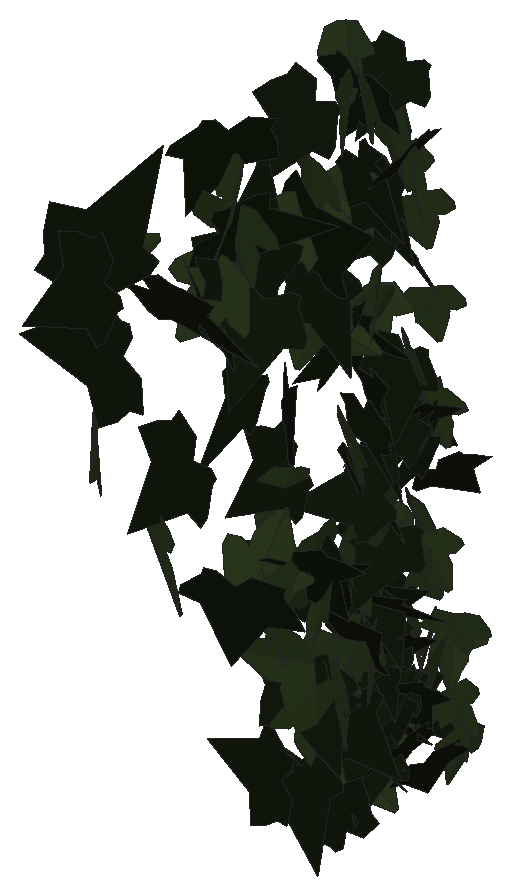
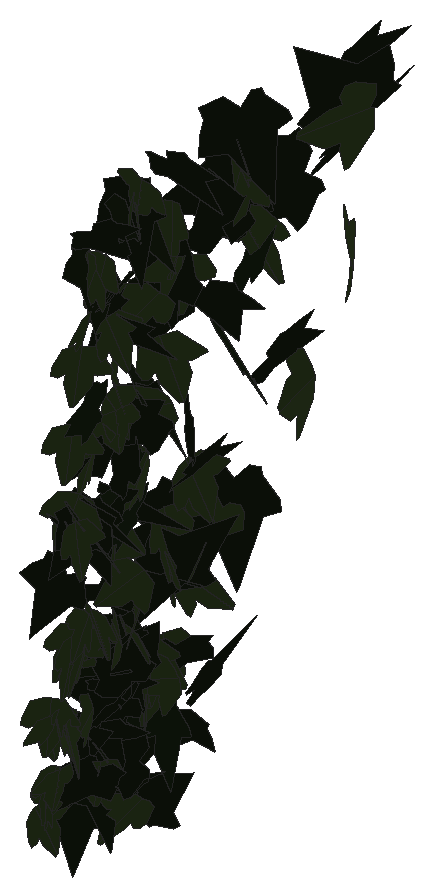
# SketchUp Ruby script. Lengths in inches.
U = 1.inch
M = Sketchup.active_model
def pt(a) = Geom::Point3d.new(a.map { |v| v * U })
def face(e, loops, mat)
  f = e.add_face(loops[0].map { |a| pt(a) })
  loops[1..].each { |l| e.add_face(l.map { |a| pt(a) }).erase! }
  f.material = f.back_material = mat if mat
  f
end
# faces: each face lists its corners as indices into pts; further lists are holes
def faces(e, pts, list, mat = nil) = list.each { |f| face(e, (f[0].is_a?(Array) ? f : [f]).map { |l| l.map { |i| pts[i] } }, mat) }
# xy, xz, yz: faces in a plane at the given z, y or x. An outline is a flat list of corners, or four numbers for a rectangle; further outlines are holes
def ring(l) = l.size == 4 ? [[l[0], l[1]], [l[2], l[1]], [l[2], l[3]], [l[0], l[3]]] : l.each_slice(2).to_a
def flat(e, list, mat, &to3) = list.each { |f| face(e, (f[0].is_a?(Array) ? f : [f]).map { |l| ring(l).map { |u, v| to3.(u, v) } }, mat) }
def xy(e, z, list, mat = nil) = flat(e, list, mat) { |x, y| [x, y, z] }
def xz(e, y, list, mat = nil) = flat(e, list, mat) { |x, z| [x, y, z] }
def yz(e, x, list, mat = nil) = flat(e, list, mat) { |y, z| [x, y, z] }
def lines(e, pts, list) = list.each { |a, b| e.add_line(pt(pts[a]), pt(pts[b])) }
# prism: a flat outline (further loops are holes) pulled along v
def prism(e, loops, v, mat = nil)
  f = face(e, loops, mat); d = Geom::Vector3d.new(v.map { |x| x * U })
  f.pushpull(f.normal.samedirection?(d) ? d.length : -d.length)
end
def box(e, o, s, mat = nil) = prism(e, [[o, [o[0] + s[0], o[1], o[2]], [o[0] + s[0], o[1] + s[1], o[2]], [o[0], o[1] + s[1], o[2]]]], [0, 0, s[2]], mat)
def at(x, y, z, deg = 0) = Geom::Transformation.translation(pt([x, y, z])) * Geom::Transformation.rotation(ORIGIN, Z_AXIS, deg.degrees)
def axes(o, x, y, z) = Geom::Transformation.new([*x, 0, *y, 0, *z, 0, *pt(o).to_a, 1])
def part(name) = M.definitions.add(name)
# library, detail: a bought-in or finely detailed component or shape, given as its bounding box
def library(name, o, s) = part(name).tap { |d| box(d.entities, o, s) }
def detail(e, o, s) = box(e.add_group.entities, o, s)
def put(e, d, t, mat = nil) = e.add_instance(d, t).tap { |i| i.material = mat if mat }
def group(e, t, mat = nil) = e.add_group.tap { |g| g.transformation = t; g.material = mat if mat }.entities
root = M.entities
M.materials.add("efeu1").color = [18, 25, 13]
M.materials.add("efeu2").color = [43, 57, 29]
c1 = part("ivyleaf_10")
p = [[0,0.5,-0.03],[-0.0625,2.02,-0.43],[-0.19,2.01,-0.46],[-0.54,1.05,-0.29],[-0.52,0.625,-0.18],[-0.83,0.76,-0.28],
  [-1.16,0.64,-0.33],[-1.15,0.33,-0.24],[-0.77,-0.39,0.02],[-0.3,-0.51,0.16],[0.04,-0.48,0.23],[-0.02,2.01,-0.4375],
  [-0.06,2.01,-0.43],[0.04,-0.49,0.23],[0.67,-0.49,0.14],[1.38,0.36,-0.2],[1.375,0.51,-0.24],[0.81,0.65,-0.19],
  [0.62,0.59,-0.15],[0.6,1.09,-0.28],[0.5,1.23,-0.31]]
faces(c1.entities,p,[[0,1,2,3,4,5,6,7,8,9,10],[11,12,0,13,14,15,16,17,18,19,20]],"efeu2")
c2 = part("ivyleaf_9")
p = [[1.54,2.16,1.25],[1.36,2.04,1.19],[-0.21,0.99,0.68],[-0.71,1.11,0.82],[-0.85,0.86,0.67],[-0.8,0.17,0.21],
  [-0.9,-0.01,0.1],[-0.67,-0.16,-0.02],[-0.08,-0.08,-0.05],[-0.03,-0.6,-0.4],[0.65,-0.88,-0.66],[0.83,-0.6,-0.49],
  [1.29,-0.42,-0.43],[1.8125,-0.07,-0.26],[1.21,0.44,0.15]]
faces(c2.entities,p,[[0,1,2,3,4,5,6,7,8,9,10,11,12,13,14]],"efeu1")
put(root,c1,axes([600.42,135.75,192.35],[-0.57947,-0.09583,-0.54206],[0.53378,0.09451,-0.58732],[0.13452,-0.78783,-0.00451]))
put(root,c2,axes([601.29,134.13,183.22],[0.15939,-0.00668,0.8756],[-0.77177,0.41934,0.14369],[-0.41362,-0.785,0.0693]))
put(root,c2,axes([600.17,135.93,185.94],[0.73929,-0.09917,0.34207],[0.33915,-0.04465,-0.74591],[0.10876,0.81337,0.00076]))
put(root,c1,axes([600.875,136.26,201.3],[-0.11468,-0.73234,0.25084],[-0.01013,-0.25213,-0.74076],[0.77404,-0.11181,0.02747]))
put(root,c1,axes([600.48,135.19,206.09],[0.75673,-0.04398,0.3091],[0.30983,0.00602,-0.75768],[0.03843,0.8174,0.02221]))
put(root,c2,axes([600.82,132.46,194.53],[-0.32847,-0.57411,0.70321],[-0.20623,-0.68108,-0.65238],[0.88406,-0.37219,0.10909]))
put(root,c1,axes([600.52,135.61,184.05],[0.26824,0.56099,0.52859],[0.23902,0.47156,-0.62176],[-0.7328,0.35917,-0.00931]))
put(root,c1,axes([600.5625,124.19,203.86],[0.0746,-0.00351,-1.25714],[0.50326,1.15412,0.02664],[1.15202,-0.50395,0.06977]))
put(root,c1,axes([600.97,132.1,194.31],[-0.17849,-0.85958,0.319],[0.01065,-0.32691,-0.87494],[0.9168,-0.16355,0.07227]))
put(root,c1,axes([600.34,134.18,188.08],[-0.33958,0.10618,-0.76231],[0.72104,-0.24756,-0.35568],[-0.26922,-0.79696,0.00892]))
put(root,c2,axes([600.39,134.69,197.75],[0.7539,0.15262,0.31025],[0.30319,0.06595,-0.76919],[-0.1662,0.81258,0.00416]))
put(root,c2,axes([601.1875,129.375,206],[0.12559,0.81604,-0.69572],[-0.07243,-0.69242,-0.82525],[-1.06991,0.14266,-0.0258]))
put(root,c1,axes([600.51,134.69,201.83],[0.49246,0.4161,0.51638],[0.38042,0.34959,-0.64449],[-0.5432,0.62205,0.01679]))
put(root,c2,axes([601.39,132.66,190.91],[0.16136,0.04894,0.94365],[-0.92224,-0.20032,0.16809],[0.20577,-0.93616,0.01336]))
put(root,c1,axes([600.89,135.32,189.9375],[0.75204,-0.43582,0.00601],[0.01492,0.01376,-0.86898],[0.4356,0.75194,0.01939]))
put(root,c1,axes([600.87,136.04,198.04],[0.30519,0.6869,-0.11948],[-0.05319,-0.1071,-0.75163],[-0.69518,0.30974,0.00506]))
put(root,c2,axes([601.36,133.27,186.28],[-0.19484,0.94153,0.12857],[-0.07206,0.11622,-0.96034],[-0.94753,-0.20245,0.0466]))
put(root,c1,axes([600.87,138.97,186.45],[0.12127,0.66909,-0.01265],[-0.00008,-0.01284,-0.67999],[-0.66921,0.12125,-0.00221]))
put(root,c2,axes([601.27,134.74,205.34],[0.58647,0.27011,-0.77571],[-0.72255,-0.28365,-0.64505],[-0.39064,0.93017,0.02856]))
put(root,c2,axes([600.67,132.57,195.53],[-0.17798,0.33647,0.88831],[0.14761,-0.88299,0.36404],[0.93836,0.20272,0.11123]))
put(root,c2,axes([601.41,134.7,204.93],[-0.50561,0.68441,-0.28331],[0.01783,-0.33167,-0.83306],[-0.74052,-0.47529,0.17338]))
put(root,c1,axes([600.45,134.44,197.9],[-0.31329,-0.15336,-0.74743],[0.75783,0.03143,-0.3241],[0.08874,-0.80983,0.12897]))
put(root,c1,axes([600.5,124.83,198.99],[-0.08943,0.09935,-1.22983],[0.473,-1.13609,-0.12617],[-1.13957,-0.47935,0.04414]))
put(root,c1,axes([600.85,136.95,185.85],[0.43736,0.59441,0.03481],[0.01938,0.02896,-0.73798],[-0.59511,0.43779,0.00155]))
put(root,c1,axes([601.24,133.2,199.09],[-0.64986,-0.57022,0.32563],[-0.14012,-0.32717,-0.85254],[0.64152,-0.64908,0.14365]))
put(root,c1,axes([601.09,137.72,194.52],[-0.11861,-0.72719,-0.02028],[0.00854,0.01915,-0.73678],[0.72742,-0.1188,0.00535]))
put(root,c1,axes([600.84,132.8125,202.08],[0.65597,0.72367,0.01641],[0.01062,0.01252,-0.97672],[-0.72378,0.65605,0.00054]))
put(root,c2,axes([600.57,137.42,199.07],[0.6371,-0.42672,0.06495],[0.04307,-0.05237,-0.76655],[0.42948,0.63826,-0.01947]))
put(root,c2,axes([600.8,124.2,204.12],[-0.46686,-0.24231,1.14678],[0.97881,0.59845,0.52493],[-0.64477,1.08393,-0.03346]))
put(root,c2,axes([601.43,135.5,200.95],[-0.82481,-0.21666,0.16799],[-0.14614,-0.10316,-0.85057],[0.23195,-0.8354,0.06146]))
put(root,c2,axes([600.74,136.28,187.96],[0.16956,-0.80811,-0.09241],[-0.02675,0.08881,-0.82567],[0.81294,0.17148,-0.0079]))
put(root,c1,axes([601.03,137.5,191.24],[-0.6172,0.34973,-0.07002],[0.05498,-0.04498,-0.70929],[-0.3524,-0.61953,0.01197]))
put(root,c1,axes([601.03,136.81,191.15],[0.67928,-0.29894,-0.04096],[-0.036,0.01989,-0.74214],[0.29958,0.68023,0.0037]))
put(root,c1,axes([601.3,128.95,201.88],[1.02623,-0.09184,-0.47066],[-0.46604,0.07092,-1.02999],[0.11298,1.12678,0.02647]))
put(root,c2,axes([600.46,135.91,188.8],[0.11426,-0.18914,0.75301],[0.74962,-0.1713,-0.15677],[0.20215,0.74212,0.15573]))
put(root,c1,axes([601.05,134.63,190.83],[-0.5381,0.68938,0.05134],[-0.01734,0.05158,-0.87434],[-0.69107,-0.53808,-0.01804]))
put(root,c1,axes([601.12,138.03,187.44],[0.3224,-0.60247,-0.07417],[-0.03645,0.06462,-0.68331],[0.60593,0.32445,-0.00164]))
put(root,c1,axes([601.0625,137.66,190.09],[-0.49479,0.50117,-0.00216],[0.00138,-0.00168,-0.70426],[-0.50117,-0.49479,0.0002]))
put(root,c2,axes([600.875,135.87,184.78],[-0.28621,-0.78529,0.08726],[0.16267,-0.14939,-0.81083],[0.7732,-0.25925,0.20289]))
put(root,c1,axes([601.13,133.75,187.9],[-0.31715,-0.75146,-0.30111],[0.10381,0.28298,-0.81553],[0.80286,-0.33344,-0.0135]))
put(root,c2,axes([601.21,136.72,204.87],[-0.55941,-0.57491,0.05908],[-0.054,-0.02987,-0.80196],[0.57541,-0.56172,-0.01783]))
put(root,c2,axes([600.53,135.18,185.34],[0.64128,-0.34646,0.28615],[0.25479,-0.13038,-0.72886],[0.37013,0.69002,0.00596]))
put(root,c2,axes([601.05,128.04,196.68],[-0.25506,-0.76369,0.73671],[-0.22915,-0.70017,-0.80515],[1.03608,-0.34287,0.00328]))
put(root,c1,axes([601.17,135.78,198.25],[0.05644,-0.71724,0.38027],[0.0236,-0.37958,-0.71944],[0.81147,0.06092,-0.00553]))
put(root,c2,axes([601.24,136.27,186.82],[-0.63447,-0.50927,-0.0238],[0.02074,0.01218,-0.81357],[0.5094,-0.6348,0.00348]))
put(root,c1,axes([600.74,136.14,190.14],[-0.05555,0.12773,-0.75309],[0.40276,-0.63668,-0.13769],[-0.64903,-0.40603,-0.02099]))
put(root,c2,axes([601.21,135.91,188.39],[-0.59629,-0.57435,-0.02227],[0.0133,0.0183,-0.82791],[0.57463,-0.59642,-0.00395]))
put(root,c1,axes([601.44,132.7,203.59],[-0.86133,0.29022,0.30649],[-0.31064,0.0357,-0.9068],[-0.28578,-0.91354,0.06193]))
put(root,c2,axes([600.85,137.07,185.87],[0.0484,-0.29496,-0.71405],[0.08231,0.71335,-0.28909],[0.76818,-0.05785,0.07596]))
put(root,c1,axes([600.96,137.34,187.98],[-0.40273,0.44585,-0.38218],[0.22974,-0.30685,-0.60007],[-0.54042,-0.4627,0.0297]))
put(root,c2,axes([601.45,132.61,205.53],[-0.93032,-0.26697,-0.1007],[0.09403,0.03737,-0.96782],[0.26939,-0.93501,-0.00993]))
put(root,c2,axes([601.7,133.67,198.1],[-0.67645,0.66652,0.01684],[-0.00823,0.01564,-0.94963],[-0.66668,-0.67648,-0.00536]))
put(root,c1,axes([600.76,126.79,195.3],[-0.682,0.68808,-0.743],[0.54477,-0.50584,-0.96849],[-0.85365,-0.87253,-0.02446]))
put(root,c2,axes([601.48,130.14,198.4],[-0.95246,0.29765,-0.41369],[0.39082,-0.13621,-0.99781],[-0.3271,-1.02945,0.01241]))
put(root,c2,axes([600.86,129.35,200.36],[-0.20453,-0.30982,1.0056],[0.21481,-1.01514,-0.26907],[1.03008,0.15018,0.25578]))
put(root,c1,axes([600.9375,130.98,191.95],[0.81918,0.43956,-0.3696],[0.31755,0.18979,0.92952],[0.47852,-0.87843,0.01588]))
put(root,c2,axes([600.74,135.65,195.75],[0.05873,-0.15285,0.76619],[0.3896,-0.66027,-0.16158],[0.67722,0.39311,0.02651]))
put(root,c2,axes([601.27,130.96,200.27],[-0.80788,-0.56282,-0.29022],[0.24835,0.15116,-0.98445],[0.58251,-0.84501,0.0172]))
put(root,c1,axes([600.98,134.72,204.91],[0.30645,-0.58251,0.55429],[0.42777,-0.38417,-0.64023],[0.68086,0.50355,0.15277]))
put(root,c1,axes([601.09,131.35,191.47],[-0.40241,0.84864,-0.31541],[0.1653,-0.27049,-0.93867],[-0.89014,-0.43388,-0.03172]))
put(root,c1,axes([601.39,134.83,205.19],[-0.67626,0.58131,0.08761],[-0.11445,0.0008,-0.88872],[-0.57663,-0.68191,0.07364]))
put(root,c1,axes([601.56,134.14,188.55],[-0.58002,-0.65861,0.2129],[-0.15332,-0.14862,-0.87745],[0.67497,-0.59972,-0.01636]))
put(root,c1,axes([601.36,137.25,200.53],[-0.51434,-0.57058,-0.10471],[0.08601,0.06339,-0.76789],[0.5737,-0.52105,0.02124]))
put(root,c2,axes([601.55,129.33,192.52],[0.69017,0.64815,-0.68048],[-0.49855,-0.46316,-0.9468],[-0.79662,0.85139,0.00298]))
put(root,c1,axes([601.26,137.04,201.88],[-0.22898,0.74611,-0.10082],[0.04723,-0.09094,-0.78024],[-0.75141,-0.23308,-0.01832]))
put(root,c2,axes([601.64,136,184.87],[-0.11842,0.79962,-0.14954],[0.02993,-0.14673,-0.8083],[-0.81293,-0.12188,-0.00798]))
put(root,c2,axes([601.51,131.125,186.05],[0.10503,-0.94989,-0.2167],[0.15393,-0.19904,0.94709],[-0.96206,-0.13554,0.12788]))
put(root,c2,axes([601.83,136.38,194.58],[-0.79579,0.02715,0.13407],[-0.13433,-0.00566,-0.79619],[-0.02583,-0.80698,0.0101]))
put(root,c2,axes([601.05,135.82,189.8],[0.09431,-0.81585,-0.18626],[0.1084,0.19777,-0.81138],[0.82979,0.06689,0.12716]))
put(root,c1,axes([601.48,129.2,203.75],[-1.12996,0.05466,-0.05608],[0.05636,0.00448,-1.13126],[-0.05437,-1.13134,-0.00719]))
put(root,c2,axes([601.65,136.59,194.52],[0.00213,0.65958,-0.47998],[0.00441,-0.47998,-0.65957],[-0.81573,-0.00087,-0.00482]))
put(root,c2,axes([601.51,135.43,187.94],[0.35174,0.77528,0.01543],[-0.02705,0.0292,-0.85055],[-0.77496,0.35086,0.0367]))
put(root,c1,axes([601.79,133.54,187.19],[0.23558,-0.29083,-0.85323],[-0.39433,0.75978,-0.36786],[0.81061,0.45413,0.06902]))
put(root,c1,axes([602.18,131.01,189.84],[0.26175,-0.01114,-1.02215],[-0.97591,0.31122,-0.2533],[0.30415,1.00819,0.0669]))
put(root,c2,axes([601.14,135.02,202.66],[0.46531,-0.625,-0.33915],[-0.1702,0.29563,-0.77833],[0.69042,0.4941,0.03669]))
put(root,c2,axes([601.82,136.1,186.32],[-0.74386,0.29825,-0.1157],[0.08906,-0.08822,-0.79997],[-0.30726,-0.74762,0.04824]))
put(root,c1,axes([601.55,137.45,197.72],[-0.59397,-0.46268,-0.06511],[0.05369,0.03703,-0.7529],[0.46414,-0.59638,0.00376]))
put(root,c1,axes([601.59,132.59,192.51],[-0.0302,-0.91844,-0.1147],[0.01392,0.11429,-0.91888],[0.92547,-0.0317,0.01008]))
put(root,c2,axes([601.59,129.81,201.69],[-0.57177,-0.56786,0.81892],[0.62656,0.52933,0.80452],[-0.77493,0.84697,0.04626]))
put(root,c2,axes([601.05,135.13,189.45],[0.79554,0.14562,0.3072],[0.24781,0.2868,-0.77769],[-0.23275,0.80312,0.22202]))
put(root,c1,axes([601.14,136.71,203.27],[0.54375,-0.38918,0.43163],[0.47411,-0.04483,-0.63768],[0.33613,0.69279,0.20121]))
put(root,c2,axes([601.47,136.125,186.41],[0.59064,0.53904,-0.10921],[-0.09387,-0.0591,-0.7994],[-0.54192,0.59774,0.01944]))
put(root,c1,axes([601.24,135.58,198.93],[0.4779,-0.45427,0.49056],[0.38114,-0.31033,-0.65866],[0.54932,0.61052,0.03022]))
put(root,c2,axes([601.19,132.68,188.26],[-0.06617,-0.79037,-0.52122],[0.14853,0.50735,-0.7882],[0.93503,-0.13652,0.08832]))
put(root,c1,axes([601.61,135.91,203.13],[-0.76893,0.19423,-0.00204],[0.00202,-0.00033,-0.79308],[-0.19423,-0.76893,-0.00017]))
put(root,c2,axes([601.34,135.35,201.96],[0.31216,-0.64426,-0.50578],[-0.24042,0.44535,-0.71567],[0.78299,0.3936,-0.01811]))
put(root,c2,axes([602.02,136.61,194.5],[-0.6615,0.43923,0.04747],[-0.04493,0.01816,-0.79398],[-0.43949,-0.66295,0.00971]))
put(root,c1,axes([601.52,134,195.2],[-0.69046,0.60608,-0.07259],[0.06895,-0.03146,-0.91848],[-0.60651,-0.69356,-0.02178]))
put(root,c1,axes([601.55,129.2,204.79],[0.78886,-0.8078,0.0551],[0.05263,-0.02561,-1.12892],[0.80796,0.79037,0.01973]))
put(root,c2,axes([601.18,134.77,193.92],[0.66127,-0.56254,-0.10977],[-0.07954,0.07591,-0.86815],[0.5676,0.66601,0.00623]))
put(root,c1,axes([601.66,137.21,189.93],[-0.0815,-0.71279,-0.30144],[0.10587,0.28999,-0.71433],[0.76663,-0.11583,0.0666]))
put(root,c1,axes([601.6875,131.9,191.82],[0.05199,-0.81421,0.59742],[0.08294,-0.59274,-0.81506],[1.00646,0.09091,0.03631]))
put(root,c1,axes([601.68,136.41,196.61],[-0.61002,0.53273,0.01084],[-0.01213,0.00259,-0.80987],[-0.5327,-0.61011,0.00602]))
put(root,c2,axes([601.56,136.47,194.43],[0.49702,0.62737,0.15242],[0.09373,0.12019,-0.80039],[-0.63878,0.50578,0.00114]))
put(root,c2,axes([601.67,132.07,191.47],[0.4711,0.86858,0.16422],[0.07713,0.14499,-0.98811],[-0.88059,0.47737,0.00131]))
put(root,c1,axes([601.71,132.51,187.89],[-0.26302,-0.95674,0.05571],[0.14516,-0.09687,-0.97836],[0.9473,-0.2508,0.16538]))
put(root,c2,axes([601.18,134.66,188.48],[-0.13654,-0.25139,0.83172],[0.58422,-0.64976,-0.10048],[0.64315,0.53686,0.26785]))
put(root,c2,axes([601.89,136.79,184.17],[0.10573,0.77979,-0.05082],[-0.03316,-0.04676,-0.78647],[-0.78074,0.10759,0.02652]))
put(root,c2,axes([601.75,135.66,191.5625],[-0.55096,-0.65377,0.02912],[-0.00749,-0.03177,-0.85484],[0.65438,-0.55081,0.01473]))
put(root,c2,axes([601.34,132.31,185.7],[-0.4745,-0.38228,-0.72656],[0.66714,0.30957,-0.59856],[0.4785,-0.81069,0.11404]))
put(root,c1,axes([601.41,135.35,188.37],[0.32433,-0.50354,0.60933],[0.44494,-0.42808,-0.59059],[0.65335,0.5415,0.09973]))
put(root,c1,axes([601.65,137.13,190.41],[-0.47299,-0.55815,-0.2835],[0.25973,0.14833,-0.72538],[0.5696,-0.53112,0.09534]))
put(root,c2,axes([601.42,132.9375,200.18],[0.18177,-0.83835,-0.36779],[-0.05984,0.36329,-0.85766],[0.91352,0.19061,0.017]))
put(root,c2,axes([601.5,133.81,186.84],[0.25923,-0.49164,-0.71685],[-0.19302,0.69682,-0.5477],[0.84755,0.30907,0.09453]))
put(root,c2,axes([600.93,133.01,201.06],[0.08092,-0.04723,1.21431],[0.83408,-0.88293,-0.08992],[0.8838,0.83758,-0.02632]))
put(root,c1,axes([601.87,134.78,192.76],[-0.1032,-0.84841,-0.28929],[0.02355,0.28853,-0.85459],[0.89606,-0.10529,-0.01086]))
put(root,c2,axes([602.07,135.57,202.88],[-0.06994,0.8345,0.0914],[-0.02202,0.08986,-0.8373],[-0.8392,-0.0719,0.01435]))
put(root,c2,axes([601.17,126.48,202.49],[1.13957,0.07045,0.1905],[0.18931,0.02482,-1.14167],[-0.07357,1.15511,0.01291]))
put(root,c2,axes([601.33,135.01,195.2],[0.47032,-0.73935,0.1343],[0.07965,-0.10849,-0.87622],[0.74722,0.47694,0.00887]))
put(root,c2,axes([601.9375,123.92,201.99],[0.33526,-1.14336,-0.47479],[0.14091,-0.45346,1.19148],[-1.22997,-0.3636,0.00708]))
put(root,c1,axes([601.55,133.37,188.08],[-0.49355,0.51709,-0.58666],[0.34419,-0.47929,-0.71201],[-0.7022,-0.59837,0.06335]))
put(root,c2,axes([601.65,136.26,196.47],[-0.08963,-0.82441,0.06829],[-0.02005,-0.0665,-0.82917],[0.82699,-0.09096,-0.0127]))
put(root,c1,axes([601.83,137.92,185.6],[-0.26751,-0.66675,-0.19208],[0.1642,0.13918,-0.71182],[0.67416,-0.29847,0.09715]))
put(root,c2,axes([601.45,128.95,203.3],[0.03642,0.49674,-1.00223],[0.0819,0.99889,0.49806],[1.11558,-0.08955,-0.00384]))
put(root,c2,axes([601.81,137.47,192.64],[0.43699,0.62088,0.10989],[0.05558,0.09525,-0.75919],[-0.62807,0.44041,0.00927]))
put(root,c1,axes([601.84,136.97,194.94],[-0.71793,-0.27757,-0.18304],[0.17136,0.06437,-0.76972],[0.28493,-0.7381,0.0017]))
put(root,c2,axes([602.54,134.09,193.62],[-0.71934,0.06382,0.52703],[-0.52854,-0.00287,-0.72105],[-0.04978,-0.89174,0.04004]))
put(root,c1,axes([601.86,138.4,185.02],[-0.56162,0.32027,-0.13788],[0.03209,-0.21283,-0.62504],[-0.34721,-0.53771,0.16527]))
put(root,c2,axes([602.14,136.67,194.01],[-0.70681,0.26897,-0.29214],[0.24796,-0.16693,-0.75361],[-0.31017,-0.74637,0.06327]))
put(root,c2,axes([601.74,131.49,192.37],[0.82423,0.61266,-0.081],[-0.05607,-0.06035,-1.02688],[-0.61544,0.826,-0.01494]))
put(root,c1,axes([601.88,137.4375,187.29],[0.30882,-0.66256,0.17446],[0.08297,-0.15379,-0.73093],[0.6801,0.31962,0.00995]))
put(root,c2,axes([601.99,123.13,204.53],[-0.30586,-0.52476,0.89834],[-0.37215,-0.81922,-0.60525],[0.97154,-0.47901,0.05098]))
put(root,c1,axes([602.01,138.39,184.32],[-0.07019,-0.6671,0.23811],[-0.01389,-0.23793,-0.6707],[0.70818,-0.07078,0.01044]))
put(root,c1,axes([601.82,132.54,191.3125],[0.79224,-0.59003,0.14227],[0.12354,-0.07228,-0.9877],[0.59424,0.80166,0.01566]))
put(root,c1,axes([602.07,137.91,187.96],[-0.65325,-0.33134,0.01624],[-0.01856,0.00068,-0.73242],[0.33122,-0.65345,-0.009]))
put(root,c1,axes([601.95,137.95,187.55],[0.19123,0.70778,-0.10833],[-0.10181,-0.08411,-0.72926],[-0.70875,0.20305,0.07553]))
